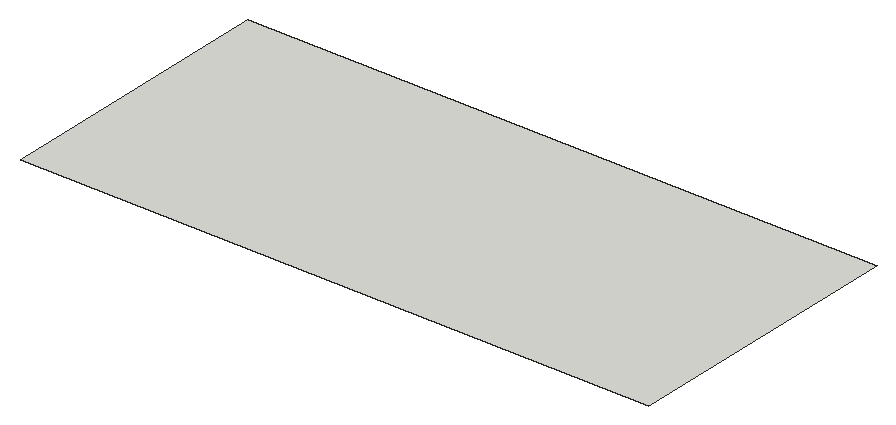
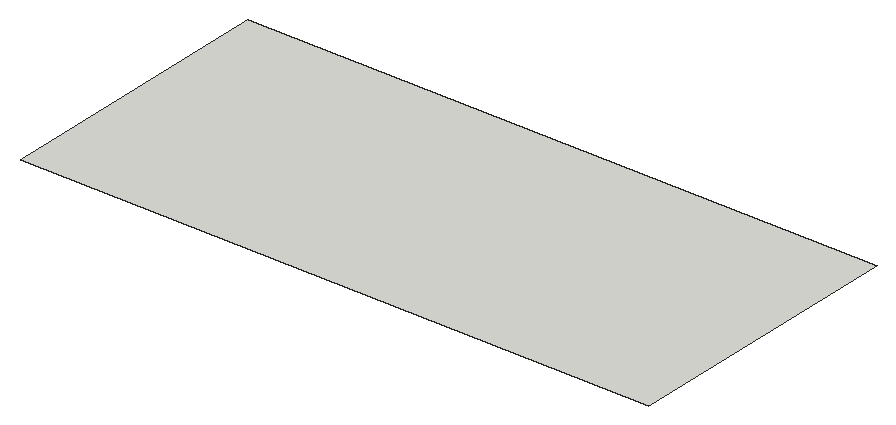
# SketchUp Ruby script. Lengths in inches.
U = 1.inch
M = Sketchup.active_model
def pt(a) = Geom::Point3d.new(a.map { |v| v * U })
def face(e, loops, mat)
  f = e.add_face(loops[0].map { |a| pt(a) })
  loops[1..].each { |l| e.add_face(l.map { |a| pt(a) }).erase! }
  f.material = f.back_material = mat if mat
  f
end
# faces: each face lists its corners as indices into pts; further lists are holes
def faces(e, pts, list, mat = nil) = list.each { |f| face(e, (f[0].is_a?(Array) ? f : [f]).map { |l| l.map { |i| pts[i] } }, mat) }
# xy, xz, yz: faces in a plane at the given z, y or x. An outline is a flat list of corners, or four numbers for a rectangle; further outlines are holes
def ring(l) = l.size == 4 ? [[l[0], l[1]], [l[2], l[1]], [l[2], l[3]], [l[0], l[3]]] : l.each_slice(2).to_a
def flat(e, list, mat, &to3) = list.each { |f| face(e, (f[0].is_a?(Array) ? f : [f]).map { |l| ring(l).map { |u, v| to3.(u, v) } }, mat) }
def xy(e, z, list, mat = nil) = flat(e, list, mat) { |x, y| [x, y, z] }
def xz(e, y, list, mat = nil) = flat(e, list, mat) { |x, z| [x, y, z] }
def yz(e, x, list, mat = nil) = flat(e, list, mat) { |y, z| [x, y, z] }
def lines(e, pts, list) = list.each { |a, b| e.add_line(pt(pts[a]), pt(pts[b])) }
# prism: a flat outline (further loops are holes) pulled along v
def prism(e, loops, v, mat = nil)
  f = face(e, loops, mat); d = Geom::Vector3d.new(v.map { |x| x * U })
  f.pushpull(f.normal.samedirection?(d) ? d.length : -d.length)
end
def box(e, o, s, mat = nil) = prism(e, [[o, [o[0] + s[0], o[1], o[2]], [o[0] + s[0], o[1] + s[1], o[2]], [o[0], o[1] + s[1], o[2]]]], [0, 0, s[2]], mat)
def at(x, y, z, deg = 0) = Geom::Transformation.translation(pt([x, y, z])) * Geom::Transformation.rotation(ORIGIN, Z_AXIS, deg.degrees)
def axes(o, x, y, z) = Geom::Transformation.new([*x, 0, *y, 0, *z, 0, *pt(o).to_a, 1])
def part(name) = M.definitions.add(name)
# library, detail: a bought-in or finely detailed component or shape, given as its bounding box
def library(name, o, s) = part(name).tap { |d| box(d.entities, o, s) }
def detail(e, o, s) = box(e.add_group.entities, o, s)
def put(e, d, t, mat = nil) = e.add_instance(d, t).tap { |i| i.material = mat if mat }
def group(e, t, mat = nil) = e.add_group.tap { |g| g.transformation = t; g.material = mat if mat }.entities
root = M.entities
xy(root,0,[[321.5,117.03,469.67,184.11]])
